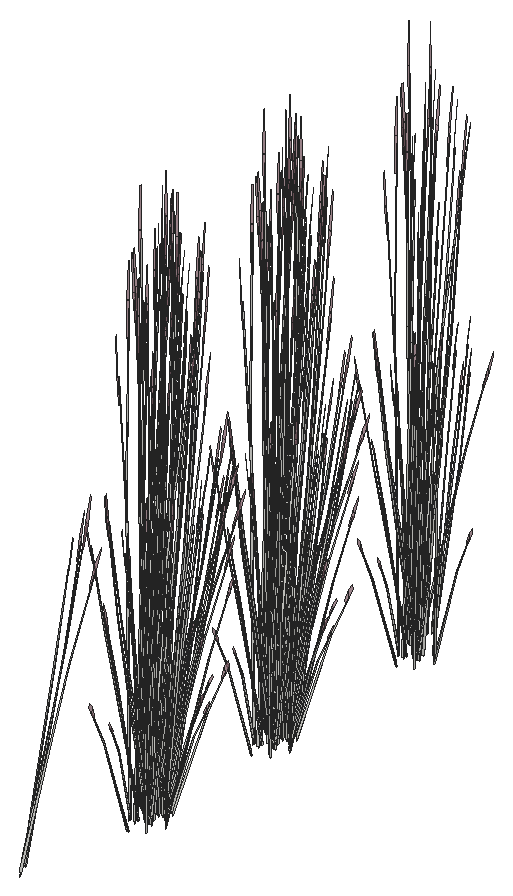
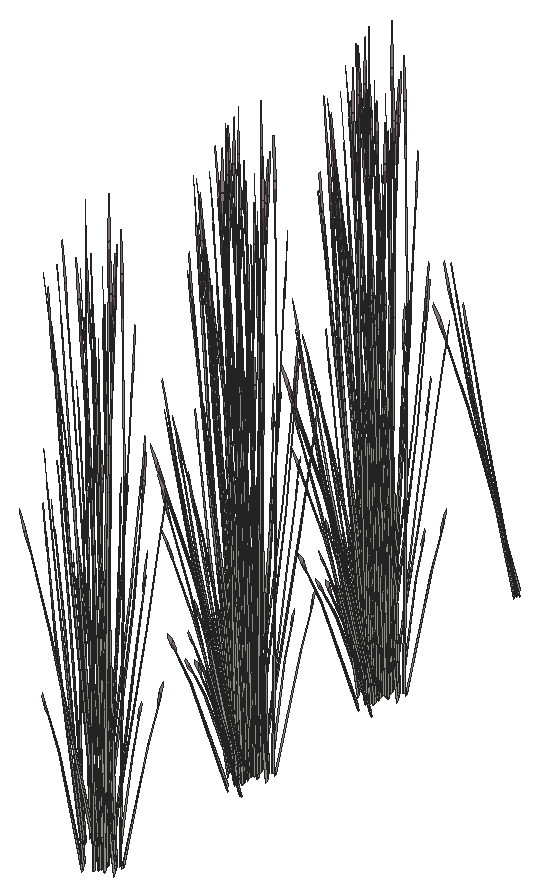
# SketchUp Ruby script. Lengths in inches.
U = 1.inch
M = Sketchup.active_model
def pt(a) = Geom::Point3d.new(a.map { |v| v * U })
def face(e, loops, mat)
  f = e.add_face(loops[0].map { |a| pt(a) })
  loops[1..].each { |l| e.add_face(l.map { |a| pt(a) }).erase! }
  f.material = f.back_material = mat if mat
  f
end
# faces: each face lists its corners as indices into pts; further lists are holes
def faces(e, pts, list, mat = nil) = list.each { |f| face(e, (f[0].is_a?(Array) ? f : [f]).map { |l| l.map { |i| pts[i] } }, mat) }
# xy, xz, yz: faces in a plane at the given z, y or x. An outline is a flat list of corners, or four numbers for a rectangle; further outlines are holes
def ring(l) = l.size == 4 ? [[l[0], l[1]], [l[2], l[1]], [l[2], l[3]], [l[0], l[3]]] : l.each_slice(2).to_a
def flat(e, list, mat, &to3) = list.each { |f| face(e, (f[0].is_a?(Array) ? f : [f]).map { |l| ring(l).map { |u, v| to3.(u, v) } }, mat) }
def xy(e, z, list, mat = nil) = flat(e, list, mat) { |x, y| [x, y, z] }
def xz(e, y, list, mat = nil) = flat(e, list, mat) { |x, z| [x, y, z] }
def yz(e, x, list, mat = nil) = flat(e, list, mat) { |y, z| [x, y, z] }
def lines(e, pts, list) = list.each { |a, b| e.add_line(pt(pts[a]), pt(pts[b])) }
# prism: a flat outline (further loops are holes) pulled along v
def prism(e, loops, v, mat = nil)
  f = face(e, loops, mat); d = Geom::Vector3d.new(v.map { |x| x * U })
  f.pushpull(f.normal.samedirection?(d) ? d.length : -d.length)
end
def box(e, o, s, mat = nil) = prism(e, [[o, [o[0] + s[0], o[1], o[2]], [o[0] + s[0], o[1] + s[1], o[2]], [o[0], o[1] + s[1], o[2]]]], [0, 0, s[2]], mat)
def at(x, y, z, deg = 0) = Geom::Transformation.translation(pt([x, y, z])) * Geom::Transformation.rotation(ORIGIN, Z_AXIS, deg.degrees)
def axes(o, x, y, z) = Geom::Transformation.new([*x, 0, *y, 0, *z, 0, *pt(o).to_a, 1])
def part(name) = M.definitions.add(name)
# library, detail: a bought-in or finely detailed component or shape, given as its bounding box
def library(name, o, s) = part(name).tap { |d| box(d.entities, o, s) }
def detail(e, o, s) = box(e.add_group.entities, o, s)
def put(e, d, t, mat = nil) = e.add_instance(d, t).tap { |i| i.material = mat if mat }
def group(e, t, mat = nil) = e.add_group.tap { |g| g.transformation = t; g.material = mat if mat }.entities
root = M.entities
M.materials.add("LightPink_Translucent").color = [144, 107, 117]
M.materials["LightPink_Translucent"].alpha = 0.75
c1 = part("blade")
p = [[2.15,0.21,22],[0,0.17,0],[0.09,0.45,0],[2.18,0.31,22],[2.29,0.31,22],[0.38,0.45,0],
  [2.48,0.24,33],[2.49,0.24,33],[2.48,0.22,33]]
faces(c1.entities,p,[[0,1,2,3],[4,5,2,3],[6,3,4,7],[8,0,3,6]])
c2 = part("seeds")
p = [[0.3,-0.1,1.38],[-0.01,-0.03,1.59],[-0.01,-0.03,0.03],[0.14,-0.07,-0.07],[0.29,-0.03,3],[0.15,0.01,3.11]]
faces(c2.entities,p,[[0,1,2,3],[1,0,4,5]],"LightPink_Translucent")
c3 = part("blade with seeds")
put(c3.entities,c1,at(0,0,0))
put(c3.entities,c2,axes([2.4,0.25,30.99],[1.5799,-0.05474,1.17369],[-0.12525,1.92788,0.29478],[-0.07173,-0.02425,1.56792]))
put(root,c3,axes([401.96,582.88,4.68],[0.34695,0.11691,-0.51099],[-0.11892,0.40083,-0.3958],[0.03181,0.16138,0.97773]))
put(root,c3,axes([402.16,582.05,3.875],[-0.08068,-0.14973,1.71376],[0.3728,-0.12606,0.13857],[0.08426,0.23506,0.73262]))
put(root,c3,axes([401.8,583.125,4.53],[-0.1064,0.35863,-0.35414],[-0.31043,-0.1046,0.4572],[0.02846,0.14439,0.87481]))
put(root,c3,axes([401.84,582.8,4.98],[0.16845,0.3792,-0.71045],[-0.34676,0.21133,0.08574],[0.03939,0.18322,1.00501]))
put(root,c3,axes([402.72,598.34,2.59],[-0.10032,0.0944,1.43002],[-0.30046,-0.16522,-0.30754],[0.05569,-0.20547,0.61141]))
put(root,c3,axes([401.98,597.83,1.49],[-0.0592,0.0168,1.76342],[-0.32738,-0.18913,-0.26939],[0.00549,-0.15776,0.30037]))
put(root,c3,axes([402.97,599.04,4.98],[0.00918,-0.43138,-0.71045],[0.38672,0.02897,0.08574],[0.04081,-0.18275,1.00501]))
put(root,c3,axes([402.3,598.35,4.53],[0.1064,-0.35863,-0.35414],[0.31043,0.1046,0.4572],[-0.02846,-0.14439,0.87481]))
put(root,c3,axes([402.53,598.82,3.875],[-0.06572,0.16029,1.71376],[-0.27569,-0.33172,0.13857],[0.12437,-0.20675,0.73262]))
put(root,c3,axes([402.35,597.59,2.77],[0.04528,0.27194,1.1486],[-0.25117,-0.15062,0.84392],[0.02703,-0.13924,0.25299]))
put(root,c3,axes([402.89,598.89,4.68],[-0.25266,-0.31335,-0.51099],[0.2669,-0.27442,-0.3958],[0.03844,-0.15921,0.97773]))
put(root,c3,axes([403.13,598.78,4.53],[0.23881,-0.24554,-0.35414],[0.22606,0.28036,0.4572],[0.0344,-0.14245,0.87481]))
put(root,c3,axes([403.43,598.63,1.49],[-0.05283,-0.03674,1.76342],[-0.13569,-0.41045,-0.26939],[0.09154,-0.11138,0.30037]))
put(root,c3,axes([403.42,599.79,4.98],[0.18436,-0.36797,-0.71045],[0.32306,0.26151,0.08574],[0.11008,-0.13332,1.00501]))
put(root,c3,axes([401.43,598.72,2.375],[-0.22066,-0.46731,0],[0.36918,-0.26061,-0.51607],[0.08408,-0.05936,1.63711]))
put(root,c3,axes([403.41,599.62,4.68],[-0.09067,-0.42583,-0.51099],[0.34336,-0.07449,-0.3958],[0.0984,-0.11438,0.97773]))
put(root,c3,axes([401.73,598.64,2.02],[0.33032,-0.23318,-0.49651],[0.19744,0.41812,0],[0.07523,-0.05311,1.57504]))
put(root,c3,axes([403.69,599.45,2.59],[-0.12609,-0.01381,1.43002],[-0.12917,-0.37055,-0.30754],[0.1549,-0.10482,0.61141]))
put(root,c3,axes([402.12,599.6,2.06],[0.23773,-0.35053,-0.62353],[0.29532,0.31785,-0.16365],[0.09526,-0.08744,1.37633]))
put(root,c3,axes([403.84,598.77,2.77],[-0.11756,0.2374,1.1486],[-0.10105,-0.31895,0.84392],[0.09709,-0.07992,0.25299]))
put(root,c3,axes([403.67,599.66,4.53],[0.30722,-0.06665,-0.35414],[0.08112,0.381,0.4572],[0.08804,-0.10234,0.87481]))
put(root,c3,axes([401.71,600.22,2.21],[0.17124,-0.42022,-0.44739],[0.35581,0.20224,0.21531],[0,-0.09687,1.43643]))
put(root,c3,axes([401.86,600.01,2.67],[-0.04113,-0.53214,-0.29095],[0.42835,-0.03218,-0.50002],[0.07543,-0.07088,1.59708]))
put(root,c3,axes([401.81,598.83,2.03],[0.32928,0.11539,-0.30978],[-0.08291,0.40636,0.30978],[0.06638,-0.04686,1.38974]))
put(root,c3,axes([401.92,600.42,2.43],[0.39767,0.22603,0.24065],[-0.19139,0.46966,0.50002],[0,-0.10827,1.60543]))
put(root,c3,axes([401.79,600.11,2.72],[-0.38326,0.02879,0.44739],[-0.03466,-0.47788,-0.21531],[0.06861,-0.04843,1.43643]))
put(root,c3,axes([403.57,600.5625,4.68],[0.09562,-0.42421,-0.51099],[0.32782,0.1454,-0.3958],[0.13199,-0.0389,0.97773]))
put(root,c3,axes([403.06,598.83,2.375],[0.22066,-0.46731,0],[0.36918,0.26061,-0.51607],[0.08408,0.05936,1.63711]))
put(root,c3,axes([401.78,600.28,2.36],[0.15345,0.52148,0.45755],[-0.43845,0.18134,0.17955],[0.00536,-0.09582,1.58856]))
put(root,c3,axes([403.92,600.68,1.98],[-0.22732,0.05597,1.41583],[-0.03618,-0.44548,0.08104],[0.15921,-0.06743,0.80566]))
put(root,c3,axes([404.34,600.29,2.26],[-0.21881,-0.29821,-0.06488],[0.23965,-0.27324,-0.29416],[0.0679,-0.01924,0.97024]))
put(root,c3,axes([402.33,600.33,2.21],[0,-0.53961,0],[0.44133,0,0],[0,0,1.79456]))
put(root,c3,axes([402.87,599.08,2.48],[-0.33032,-0.23318,0.49651],[0.19744,-0.41812,0],[0.07523,0.05311,1.57504]))
put(root,c3,axes([403.51,600.72,4.98],[0.31014,-0.20596,-0.71045],[0.17284,0.42397,0.08574],[0.14985,-0.04816,1.00501]))
put(root,c3,axes([402.12,599.99,2.36],[-0.29264,0.42323,0.45755],[-0.34767,-0.3736,0.17955],[0.07055,-0.04224,1.58856]))
put(root,c3,axes([401.61,599.29,2.47],[-0.10196,0.46348,0.17642],[-0.3731,-0.13116,0.35086],[0.06445,-0.00226,1.60407]))
put(root,c3,axes([401.46,599.66,1.59],[-0.3474,0.18671,1.28929],[-0.11057,-0.53572,0.50096],[0.21332,0.00891,1.46642]))
put(root,c3,axes([402.39,599.8,2.62],[0.06809,-0.4162,0.1448],[0.33266,0.07225,-0.41347],[0.06054,0.04274,1.26744]))
put(root,c3,axes([404.17,600.39,1.49],[-0.01845,-0.0708,1.76342],[0.12793,-0.41416,-0.26939],[0.12905,-0.00596,0.30037]))
put(root,c3,axes([402.25,599.91,2.72],[-0.21202,-0.39143,0.44739],[0.32115,-0.27564,-0.21531],[0.06861,0.04843,1.43643]))
put(root,c3,axes([402.36,599.9375,2.67],[0.35635,-0.30962,-0.29095],[0.23697,0.43749,-0.50002],[0.08792,0.04443,1.59708]))
put(root,c3,axes([403.78,600.76,4.53],[0.29332,0.1301,-0.35414],[-0.08555,0.37955,0.4572],[0.11809,-0.0348,0.87481]))
put(root,c3,axes([403.26,599.12,2.02],[0.33032,0.23318,-0.49651],[-0.19744,0.41812,0],[0.07523,0.05311,1.57504]))
put(root,c3,axes([402.63,600.45,2.21],[0.39487,0,0],[0,0.48281,0],[0,0,1.78407]))
put(root,c3,axes([402.74,599.3125,2.47],[-0.37926,0.12378,0.17642],[-0.09365,-0.46065,0.35086],[0.03382,0.06712,1.60407]))
put(root,c3,axes([402.98,600.29,3.875],[-0.14639,0.01056,1.71376],[0.09712,-0.45778,0.13857],[0.20862,0.02831,0.73262]))
put(root,c3,axes([403.17,599.29,2.03],[0.08291,0.40636,-0.30978],[-0.32928,0.11539,0.30978],[0.06638,0.04686,1.38974]))
put(root,c3,axes([402.5,600.2,2.38],[-0.44609,-0.09826,0.49198],[0.09078,-0.55493,0.19306],[0.06519,0.05359,1.70813]))
put(root,c3,axes([402.15,601.57,2.2],[-0.11516,-0.40207,0],[0.32884,-0.1408,0],[0,0,1.54371]))
put(root,c3,axes([402.58,601.51,2.18],[0.37054,-0.15823,-0.19198],[0.1302,0.45581,0.00008],[0.0409,-0.01749,1.73897]))
put(root,c3,axes([402.62,600.65,2.21],[0.24637,0.30123,0],[-0.24637,0.30123,0],[0,0,1.69266]))
put(root,c3,axes([403.29,600.52,2.47],[-0.2773,-0.3397,0.17642],[0.27945,-0.32949,0.35086],[-0.03063,0.06937,1.60407]))
put(root,c3,axes([402.78,600.01,2.06],[0.36714,0.07646,-0.62353],[-0.07747,0.47163,-0.16365],[0.10956,0.05715,1.37633]))
put(root,c3,axes([404.4,600.83,2.77],[-0.21807,0.07699,1.1486],[0.10265,-0.31819,0.84392],[0.11568,0.02177,0.25299]))
put(root,c3,axes([402.62,600.3,2.72],[0.17124,-0.42022,0.44739],[0.35581,0.20224,-0.21531],[0,0.09687,1.43643]))
put(root,c3,axes([402.55,600.54,2.29],[0,0.53934,-0.05637],[-0.44133,0,0],[0,0.01695,1.79368]))
put(root,c3,axes([402.58,600.16,2.21],[0.21202,0.39143,-0.44739],[-0.32115,0.27564,0.21531],[0.06861,0.04843,1.43643]))
put(root,c3,axes([404.02,601.8125,3.93],[-0.06755,-0.39203,-0.03492],[0.31928,-0.09013,-0.15832],[0.06667,0.02485,0.52218]))
put(root,c3,axes([403.52,600.53,2.48],[0,-0.46636,0.49651],[0.39487,0,0],[0,0.10622,1.57504]))
put(root,c3,axes([402.77,600.4,2.62],[0.32884,-0.136,0.1448],[0.11516,0.38837,-0.41347],[0,0.08547,1.26744]))
put(root,c3,axes([403.99,601.34,2.59],[-0.085,-0.1147,1.43002],[0.1106,-0.37943,-0.30754],[0.17198,0.0514,0.61141]))
put(root,c3,axes([402.47,601.76,2.2],[0.35581,0.20937,0],[-0.17124,0.43505,0],[0,0,1.74954]))
put(root,c3,axes([403.21,601.57,4.98],[0.35281,0.01123,-0.71045],[-0.0237,0.47284,0.08574],[0.14947,0.0499,1.00501]))
put(root,c3,axes([402.8125,601.95,2.48],[0.33032,-0.23318,0.49651],[0.19744,0.41812,0],[-0.07523,0.05311,1.57504]))
put(root,c3,axes([402.34,601.58,2.29],[0.15345,0.53576,-0.06012],[-0.43845,0.18773,0],[0.00536,0.01871,1.72173]))
put(root,c3,axes([403.78,600.61,2.375],[0.44133,0,0],[0,0.52122,-0.51607],[0,0.11871,1.63711]))
put(root,c3,axes([403.61,600.88,2.2],[-0.44111,-0.00373,-0.04976],[0,-0.52122,0.49943],[-0.01386,0.11865,1.58352]))
put(root,c3,axes([402.65,600.43,2.67],[0.39748,0.22252,-0.29095],[-0.19139,0.46966,-0.50002],[0.01249,0.11531,1.59708]))
put(root,c3,axes([403.42,601.77,4.53],[0.20082,0.29199,-0.35414],[-0.2293,0.2764,0.4572],[0.1165,0.04206,0.87481]))
put(root,c3,axes([403.52,600.96,2.03],[-0.24637,0.29097,-0.30978],[-0.24637,-0.29097,0.30978],[0,0.09372,1.38974]))
put(root,c3,axes([402.61,600.78,2.21],[-0.17124,0.42022,-0.44739],[-0.35581,-0.20224,0.21531],[0,0.09687,1.43643]))
put(root,c3,axes([402.62,601.98,2.33],[0.44186,0.15158,0.30756],[-0.11054,0.54181,-0.36492],[-0.07313,0.06781,1.64885]))
put(root,c3,axes([403.6875,600.97,2.02],[0,0.46636,-0.49651],[-0.39487,0,0],[0,0.10622,1.57504]))
put(root,c3,axes([402.7,601.02,3.875],[-0.1311,-0.08035,1.71376],[0.27131,-0.33708,0.13857],[0.16909,0.15206,0.73262]))
put(root,c3,axes([403.18,601.94,2.77],[-0.19872,-0.13409,1.1486],[0.2566,-0.13625,0.84392],[0.06921,0.11541,0.25299]))
put(root,c3,axes([403.24,602.43,1.49],[0.02571,-0.06733,1.76342],[0.32373,-0.19829,-0.26939],[0.09815,0.10263,0.30037]))
put(root,c3,axes([402.8125,600.9,2.09],[0.12941,0.42699,-0.69212],[-0.37279,0.15378,-0.18165],[0.0143,0.14459,1.52773]))
put(root,c3,axes([402.74,602.12,4.68],[0.34827,-0.11086,-0.51099],[0.06092,0.41983,-0.3958],[0.09354,0.12031,0.97773]))
put(root,c3,axes([403.22,602.55,2.67],[-0.22633,-0.01463,1.0506],[0.14947,-0.31064,0.58006],[0.08941,0.11036,0.8241]))
put(root,c3,axes([402.48,601.79,2.59],[0.00623,-0.15459,1.43002],[0.29764,-0.17268,-0.30754],[0.09188,0.18503,0.61141]))
put(root,c3,axes([401.73,602.42,1.49],[0.05712,-0.02538,1.76342],[0.34359,0.13968,-0.26939],[0.01005,0.15742,0.30037]))
put(root,c3,axes([401.96,602.31,4.68],[0.34695,0.11691,-0.51099],[-0.11892,0.40083,-0.3958],[0.03181,0.16138,0.97773]))
put(root,c3,axes([402.16,601.49,3.875],[-0.08068,-0.14973,1.71376],[0.3728,-0.12606,0.13857],[0.08426,0.23506,0.73262]))
put(root,c3,axes([401.8,602.5625,4.53],[-0.1064,0.35863,-0.35414],[-0.31043,-0.1046,0.4572],[0.02846,0.14439,0.87481]))
put(root,c3,axes([401.84,602.24,4.98],[0.16845,0.3792,-0.71045],[-0.34676,0.21133,0.08574],[0.03939,0.18322,1.00501]))
put(root,c3,axes([402.72,615.92,2.59],[-0.10032,0.0944,1.43002],[-0.30046,-0.16522,-0.30754],[0.05569,-0.20547,0.61141]))
put(root,c3,axes([401.98,615.41,1.49],[-0.0592,0.0168,1.76342],[-0.32738,-0.18913,-0.26939],[0.00549,-0.15776,0.30037]))
put(root,c3,axes([402.97,616.62,4.98],[0.00918,-0.43138,-0.71045],[0.38672,0.02897,0.08574],[0.04081,-0.18275,1.00501]))
put(root,c3,axes([402.3,615.93,4.53],[0.1064,-0.35863,-0.35414],[0.31043,0.1046,0.4572],[-0.02846,-0.14439,0.87481]))
put(root,c3,axes([402.53,616.4,3.875],[-0.06572,0.16029,1.71376],[-0.27569,-0.33172,0.13857],[0.12437,-0.20675,0.73262]))
put(root,c3,axes([402.35,615.17,2.77],[0.04528,0.27194,1.1486],[-0.25117,-0.15062,0.84392],[0.02703,-0.13924,0.25299]))
put(root,c3,axes([402.89,616.48,4.68],[-0.25266,-0.31335,-0.51099],[0.2669,-0.27442,-0.3958],[0.03844,-0.15921,0.97773]))
put(root,c3,axes([403.13,616.36,4.53],[0.23881,-0.24554,-0.35414],[0.22606,0.28036,0.4572],[0.0344,-0.14245,0.87481]))
put(root,c3,axes([403.43,616.21,1.49],[-0.05283,-0.03674,1.76342],[-0.13569,-0.41045,-0.26939],[0.09154,-0.11138,0.30037]))
put(root,c3,axes([403.42,617.37,4.98],[0.18436,-0.36797,-0.71045],[0.32306,0.26151,0.08574],[0.11008,-0.13332,1.00501]))
put(root,c3,axes([401.43,616.3,2.375],[-0.22066,-0.46731,0],[0.36918,-0.26061,-0.51607],[0.08408,-0.05936,1.63711]))
put(root,c3,axes([403.41,617.2,4.68],[-0.09067,-0.42583,-0.51099],[0.34336,-0.07449,-0.3958],[0.0984,-0.11438,0.97773]))
put(root,c3,axes([401.73,616.23,2.02],[0.33032,-0.23318,-0.49651],[0.19744,0.41812,0],[0.07523,-0.05311,1.57504]))
put(root,c3,axes([403.69,617.03,2.59],[-0.12609,-0.01381,1.43002],[-0.12917,-0.37055,-0.30754],[0.1549,-0.10482,0.61141]))
put(root,c3,axes([402.12,617.18,2.06],[0.23773,-0.35053,-0.62353],[0.29532,0.31785,-0.16365],[0.09526,-0.08744,1.37633]))
put(root,c3,axes([403.84,616.35,2.77],[-0.11756,0.2374,1.1486],[-0.10105,-0.31895,0.84392],[0.09709,-0.07992,0.25299]))
put(root,c3,axes([403.67,617.24,4.53],[0.30722,-0.06665,-0.35414],[0.08112,0.381,0.4572],[0.08804,-0.10234,0.87481]))
put(root,c3,axes([401.71,617.8,2.21],[0.17124,-0.42022,-0.44739],[0.35581,0.20224,0.21531],[0,-0.09687,1.43643]))
put(root,c3,axes([401.86,617.59,2.67],[-0.04113,-0.53214,-0.29095],[0.42835,-0.03218,-0.50002],[0.07543,-0.07088,1.59708]))
put(root,c3,axes([401.81,616.41,2.03],[0.32928,0.11539,-0.30978],[-0.08291,0.40636,0.30978],[0.06638,-0.04686,1.38974]))
put(root,c3,axes([401.92,618.01,2.43],[0.39767,0.22603,0.24065],[-0.19139,0.46966,0.50002],[0,-0.10827,1.60543]))
put(root,c3,axes([401.79,617.69,2.72],[-0.38326,0.02879,0.44739],[-0.03466,-0.47788,-0.21531],[0.06861,-0.04843,1.43643]))
put(root,c3,axes([403.57,618.14,4.68],[0.09562,-0.42421,-0.51099],[0.32782,0.1454,-0.3958],[0.13199,-0.0389,0.97773]))
put(root,c3,axes([403.06,616.42,2.375],[0.22066,-0.46731,0],[0.36918,0.26061,-0.51607],[0.08408,0.05936,1.63711]))
put(root,c3,axes([401.78,617.86,2.36],[0.15345,0.52148,0.45755],[-0.43845,0.18134,0.17955],[0.00536,-0.09582,1.58856]))
put(root,c3,axes([403.92,618.26,1.98],[-0.22732,0.05597,1.41583],[-0.03618,-0.44548,0.08104],[0.15921,-0.06743,0.80566]))
put(root,c3,axes([404.34,617.87,2.26],[-0.21881,-0.29821,-0.06488],[0.23965,-0.27324,-0.29416],[0.0679,-0.01924,0.97024]))
put(root,c3,axes([402.33,617.91,2.21],[0,-0.53961,0],[0.44133,0,0],[0,0,1.79456]))
put(root,c3,axes([402.87,616.66,2.48],[-0.33032,-0.23318,0.49651],[0.19744,-0.41812,0],[0.07523,0.05311,1.57504]))
put(root,c3,axes([403.51,618.3,4.98],[0.31014,-0.20596,-0.71045],[0.17284,0.42397,0.08574],[0.14985,-0.04816,1.00501]))
put(root,c3,axes([402.12,617.57,2.36],[-0.29264,0.42323,0.45755],[-0.34767,-0.3736,0.17955],[0.07055,-0.04224,1.58856]))
put(root,c3,axes([401.61,616.87,2.47],[-0.10196,0.46348,0.17642],[-0.3731,-0.13116,0.35086],[0.06445,-0.00226,1.60407]))
put(root,c3,axes([401.46,617.25,1.59],[-0.3474,0.18671,1.28929],[-0.11057,-0.53572,0.50096],[0.21332,0.00891,1.46642]))
put(root,c3,axes([402.39,617.39,2.62],[0.06809,-0.4162,0.1448],[0.33266,0.07225,-0.41347],[0.06054,0.04274,1.26744]))
put(root,c3,axes([404.17,617.97,1.49],[-0.01845,-0.0708,1.76342],[0.12793,-0.41416,-0.26939],[0.12905,-0.00596,0.30037]))
put(root,c3,axes([402.25,617.5,2.72],[-0.21202,-0.39143,0.44739],[0.32115,-0.27564,-0.21531],[0.06861,0.04843,1.43643]))
put(root,c3,axes([402.36,617.52,2.67],[0.35635,-0.30962,-0.29095],[0.23697,0.43749,-0.50002],[0.08792,0.04443,1.59708]))
put(root,c3,axes([403.78,618.34,4.53],[0.29332,0.1301,-0.35414],[-0.08555,0.37955,0.4572],[0.11809,-0.0348,0.87481]))
put(root,c3,axes([403.26,616.7,2.02],[0.33032,0.23318,-0.49651],[-0.19744,0.41812,0],[0.07523,0.05311,1.57504]))
put(root,c3,axes([402.63,618.03,2.21],[0.39487,0,0],[0,0.48281,0],[0,0,1.78407]))
put(root,c3,axes([402.74,616.9,2.47],[-0.37926,0.12378,0.17642],[-0.09365,-0.46065,0.35086],[0.03382,0.06712,1.60407]))
put(root,c3,axes([402.98,617.87,3.875],[-0.14639,0.01056,1.71376],[0.09712,-0.45778,0.13857],[0.20862,0.02831,0.73262]))
put(root,c3,axes([403.17,616.87,2.03],[0.08291,0.40636,-0.30978],[-0.32928,0.11539,0.30978],[0.06638,0.04686,1.38974]))
put(root,c3,axes([402.5,617.78,2.38],[-0.44609,-0.09826,0.49198],[0.09078,-0.55493,0.19306],[0.06519,0.05359,1.70813]))
put(root,c3,axes([402.15,619.15,2.2],[-0.11516,-0.40207,0],[0.32884,-0.1408,0],[0,0,1.54371]))
put(root,c3,axes([402.58,619.1,2.18],[0.37054,-0.15823,-0.19198],[0.1302,0.45581,0.00008],[0.0409,-0.01749,1.73897]))
put(root,c3,axes([402.62,618.24,2.21],[0.24637,0.30123,0],[-0.24637,0.30123,0],[0,0,1.69266]))
put(root,c3,axes([403.29,618.1,2.47],[-0.2773,-0.3397,0.17642],[0.27945,-0.32949,0.35086],[-0.03063,0.06937,1.60407]))
put(root,c3,axes([402.78,617.59,2.06],[0.36714,0.07646,-0.62353],[-0.07747,0.47163,-0.16365],[0.10956,0.05715,1.37633]))
put(root,c3,axes([404.4,618.42,2.77],[-0.21807,0.07699,1.1486],[0.10265,-0.31819,0.84392],[0.11568,0.02177,0.25299]))
put(root,c3,axes([402.62,617.88,2.72],[0.17124,-0.42022,0.44739],[0.35581,0.20224,-0.21531],[0,0.09687,1.43643]))
put(root,c3,axes([402.55,618.125,2.29],[0,0.53934,-0.05637],[-0.44133,0,0],[0,0.01695,1.79368]))
put(root,c3,axes([402.58,617.74,2.21],[0.21202,0.39143,-0.44739],[-0.32115,0.27564,0.21531],[0.06861,0.04843,1.43643]))
put(root,c3,axes([404.02,619.4,3.93],[-0.06755,-0.39203,-0.03492],[0.31928,-0.09013,-0.15832],[0.06667,0.02485,0.52218]))
put(root,c3,axes([403.52,618.12,2.48],[0,-0.46636,0.49651],[0.39487,0,0],[0,0.10622,1.57504]))
put(root,c3,axes([402.77,617.98,2.62],[0.32884,-0.136,0.1448],[0.11516,0.38837,-0.41347],[0,0.08547,1.26744]))
put(root,c3,axes([403.99,618.93,2.59],[-0.085,-0.1147,1.43002],[0.1106,-0.37943,-0.30754],[0.17198,0.0514,0.61141]))
put(root,c3,axes([402.47,619.34,2.2],[0.35581,0.20937,0],[-0.17124,0.43505,0],[0,0,1.74954]))
put(root,c3,axes([403.21,619.16,4.98],[0.35281,0.01123,-0.71045],[-0.0237,0.47284,0.08574],[0.14947,0.0499,1.00501]))
put(root,c3,axes([402.8125,619.54,2.48],[0.33032,-0.23318,0.49651],[0.19744,0.41812,0],[-0.07523,0.05311,1.57504]))
put(root,c3,axes([402.34,619.17,2.29],[0.15345,0.53576,-0.06012],[-0.43845,0.18773,0],[0.00536,0.01871,1.72173]))
put(root,c3,axes([403.78,618.2,2.375],[0.44133,0,0],[0,0.52122,-0.51607],[0,0.11871,1.63711]))
put(root,c3,axes([403.61,618.46,2.2],[-0.44111,-0.00373,-0.04976],[0,-0.52122,0.49943],[-0.01386,0.11865,1.58352]))
put(root,c3,axes([402.65,618.01,2.67],[0.39748,0.22252,-0.29095],[-0.19139,0.46966,-0.50002],[0.01249,0.11531,1.59708]))
put(root,c3,axes([403.42,619.35,4.53],[0.20082,0.29199,-0.35414],[-0.2293,0.2764,0.4572],[0.1165,0.04206,0.87481]))
put(root,c3,axes([403.52,618.54,2.03],[-0.24637,0.29097,-0.30978],[-0.24637,-0.29097,0.30978],[0,0.09372,1.38974]))
put(root,c3,axes([402.61,618.36,2.21],[-0.17124,0.42022,-0.44739],[-0.35581,-0.20224,0.21531],[0,0.09687,1.43643]))
put(root,c3,axes([402.62,619.57,2.33],[0.44186,0.15158,0.30756],[-0.11054,0.54181,-0.36492],[-0.07313,0.06781,1.64885]))
put(root,c3,axes([403.6875,618.55,2.02],[0,0.46636,-0.49651],[-0.39487,0,0],[0,0.10622,1.57504]))
put(root,c3,axes([402.7,618.6,3.875],[-0.1311,-0.08035,1.71376],[0.27131,-0.33708,0.13857],[0.16909,0.15206,0.73262]))
put(root,c3,axes([403.18,619.52,2.77],[-0.19872,-0.13409,1.1486],[0.2566,-0.13625,0.84392],[0.06921,0.11541,0.25299]))
put(root,c3,axes([403.24,620.02,1.49],[0.02571,-0.06733,1.76342],[0.32373,-0.19829,-0.26939],[0.09815,0.10263,0.30037]))
put(root,c3,axes([402.8125,618.49,2.09],[0.12941,0.42699,-0.69212],[-0.37279,0.15378,-0.18165],[0.0143,0.14459,1.52773]))
put(root,c3,axes([402.74,619.7,4.68],[0.34827,-0.11086,-0.51099],[0.06092,0.41983,-0.3958],[0.09354,0.12031,0.97773]))
put(root,c3,axes([403.22,620.13,2.67],[-0.22633,-0.01463,1.0506],[0.14947,-0.31064,0.58006],[0.08941,0.11036,0.8241]))
put(root,c3,axes([402.48,619.375,2.59],[0.00623,-0.15459,1.43002],[0.29764,-0.17268,-0.30754],[0.09188,0.18503,0.61141]))
put(root,c3,axes([401.73,620,1.49],[0.05712,-0.02538,1.76342],[0.34359,0.13968,-0.26939],[0.01005,0.15742,0.30037]))
put(root,c3,axes([401.96,619.9,4.68],[0.34695,0.11691,-0.51099],[-0.11892,0.40083,-0.3958],[0.03181,0.16138,0.97773]))
put(root,c3,axes([402.16,619.07,3.875],[-0.08068,-0.14973,1.71376],[0.3728,-0.12606,0.13857],[0.08426,0.23506,0.73262]))
put(root,c3,axes([401.8,620.14,4.53],[-0.1064,0.35863,-0.35414],[-0.31043,-0.1046,0.4572],[0.02846,0.14439,0.87481]))
put(root,c3,axes([401.84,619.82,4.98],[0.16845,0.3792,-0.71045],[-0.34676,0.21133,0.08574],[0.03939,0.18322,1.00501]))
put(root,c3,axes([402.72,636.46,2.59],[-0.10032,0.0944,1.43002],[-0.30046,-0.16522,-0.30754],[0.05569,-0.20547,0.61141]))
put(root,c3,axes([401.98,635.94,1.49],[-0.0592,0.0168,1.76342],[-0.32738,-0.18913,-0.26939],[0.00549,-0.15776,0.30037]))
put(root,c3,axes([402.97,637.16,4.98],[0.00918,-0.43138,-0.71045],[0.38672,0.02897,0.08574],[0.04081,-0.18275,1.00501]))
put(root,c3,axes([402.3,636.46,4.53],[0.1064,-0.35863,-0.35414],[0.31043,0.1046,0.4572],[-0.02846,-0.14439,0.87481]))
put(root,c3,axes([402.53,636.9375,3.875],[-0.06572,0.16029,1.71376],[-0.27569,-0.33172,0.13857],[0.12437,-0.20675,0.73262]))
put(root,c3,axes([402.35,635.71,2.77],[0.04528,0.27194,1.1486],[-0.25117,-0.15062,0.84392],[0.02703,-0.13924,0.25299]))
put(root,c3,axes([402.89,637.01,4.68],[-0.25266,-0.31335,-0.51099],[0.2669,-0.27442,-0.3958],[0.03844,-0.15921,0.97773]))
put(root,c3,axes([403.13,636.9,4.53],[0.23881,-0.24554,-0.35414],[0.22606,0.28036,0.4572],[0.0344,-0.14245,0.87481]))
put(root,c3,axes([403.43,636.75,1.49],[-0.05283,-0.03674,1.76342],[-0.13569,-0.41045,-0.26939],[0.09154,-0.11138,0.30037]))
put(root,c3,axes([403.42,637.91,4.98],[0.18436,-0.36797,-0.71045],[0.32306,0.26151,0.08574],[0.11008,-0.13332,1.00501]))
put(root,c3,axes([401.43,636.83,2.375],[-0.22066,-0.46731,0],[0.36918,-0.26061,-0.51607],[0.08408,-0.05936,1.63711]))
put(root,c3,axes([403.41,637.73,4.68],[-0.09067,-0.42583,-0.51099],[0.34336,-0.07449,-0.3958],[0.0984,-0.11438,0.97773]))
put(root,c3,axes([401.73,636.76,2.02],[0.33032,-0.23318,-0.49651],[0.19744,0.41812,0],[0.07523,-0.05311,1.57504]))
put(root,c3,axes([403.69,637.57,2.59],[-0.12609,-0.01381,1.43002],[-0.12917,-0.37055,-0.30754],[0.1549,-0.10482,0.61141]))
put(root,c3,axes([402.12,637.72,2.06],[0.23773,-0.35053,-0.62353],[0.29532,0.31785,-0.16365],[0.09526,-0.08744,1.37633]))
put(root,c3,axes([403.84,636.89,2.77],[-0.11756,0.2374,1.1486],[-0.10105,-0.31895,0.84392],[0.09709,-0.07992,0.25299]))
put(root,c3,axes([403.67,637.78,4.53],[0.30722,-0.06665,-0.35414],[0.08112,0.381,0.4572],[0.08804,-0.10234,0.87481]))
put(root,c3,axes([401.71,638.33,2.21],[0.17124,-0.42022,-0.44739],[0.35581,0.20224,0.21531],[0,-0.09687,1.43643]))
put(root,c3,axes([401.86,638.125,2.67],[-0.04113,-0.53214,-0.29095],[0.42835,-0.03218,-0.50002],[0.07543,-0.07088,1.59708]))
put(root,c3,axes([401.81,636.95,2.03],[0.32928,0.11539,-0.30978],[-0.08291,0.40636,0.30978],[0.06638,-0.04686,1.38974]))
put(root,c3,axes([401.92,638.54,2.43],[0.39767,0.22603,0.24065],[-0.19139,0.46966,0.50002],[0,-0.10827,1.60543]))
put(root,c3,axes([401.79,638.23,2.72],[-0.38326,0.02879,0.44739],[-0.03466,-0.47788,-0.21531],[0.06861,-0.04843,1.43643]))
put(root,c3,axes([403.57,638.68,4.68],[0.09562,-0.42421,-0.51099],[0.32782,0.1454,-0.3958],[0.13199,-0.0389,0.97773]))
put(root,c3,axes([403.06,636.95,2.375],[0.22066,-0.46731,0],[0.36918,0.26061,-0.51607],[0.08408,0.05936,1.63711]))
put(root,c3,axes([401.78,638.4,2.36],[0.15345,0.52148,0.45755],[-0.43845,0.18134,0.17955],[0.00536,-0.09582,1.58856]))
put(root,c3,axes([403.92,638.8,1.98],[-0.22732,0.05597,1.41583],[-0.03618,-0.44548,0.08104],[0.15921,-0.06743,0.80566]))
put(root,c3,axes([404.34,638.4,2.26],[-0.21881,-0.29821,-0.06488],[0.23965,-0.27324,-0.29416],[0.0679,-0.01924,0.97024]))
put(root,c3,axes([402.33,638.44,2.21],[0,-0.53961,0],[0.44133,0,0],[0,0,1.79456]))
put(root,c3,axes([402.87,637.2,2.48],[-0.33032,-0.23318,0.49651],[0.19744,-0.41812,0],[0.07523,0.05311,1.57504]))
put(root,c3,axes([403.51,638.83,4.98],[0.31014,-0.20596,-0.71045],[0.17284,0.42397,0.08574],[0.14985,-0.04816,1.00501]))
put(root,c3,axes([402.12,638.1,2.36],[-0.29264,0.42323,0.45755],[-0.34767,-0.3736,0.17955],[0.07055,-0.04224,1.58856]))
put(root,c3,axes([401.61,637.41,2.47],[-0.10196,0.46348,0.17642],[-0.3731,-0.13116,0.35086],[0.06445,-0.00226,1.60407]))
put(root,c3,axes([401.46,637.78,1.59],[-0.3474,0.18671,1.28929],[-0.11057,-0.53572,0.50096],[0.21332,0.00891,1.46642]))
put(root,c3,axes([402.39,637.92,2.62],[0.06809,-0.4162,0.1448],[0.33266,0.07225,-0.41347],[0.06054,0.04274,1.26744]))
put(root,c3,axes([404.17,638.51,1.49],[-0.01845,-0.0708,1.76342],[0.12793,-0.41416,-0.26939],[0.12905,-0.00596,0.30037]))
put(root,c3,axes([402.25,638.03,2.72],[-0.21202,-0.39143,0.44739],[0.32115,-0.27564,-0.21531],[0.06861,0.04843,1.43643]))
put(root,c3,axes([402.36,638.06,2.67],[0.35635,-0.30962,-0.29095],[0.23697,0.43749,-0.50002],[0.08792,0.04443,1.59708]))
put(root,c3,axes([403.78,638.87,4.53],[0.29332,0.1301,-0.35414],[-0.08555,0.37955,0.4572],[0.11809,-0.0348,0.87481]))
put(root,c3,axes([403.26,637.23,2.02],[0.33032,0.23318,-0.49651],[-0.19744,0.41812,0],[0.07523,0.05311,1.57504]))
put(root,c3,axes([402.63,638.5625,2.21],[0.39487,0,0],[0,0.48281,0],[0,0,1.78407]))
put(root,c3,axes([402.74,637.43,2.47],[-0.37926,0.12378,0.17642],[-0.09365,-0.46065,0.35086],[0.03382,0.06712,1.60407]))
put(root,c3,axes([402.98,638.4,3.875],[-0.14639,0.01056,1.71376],[0.09712,-0.45778,0.13857],[0.20862,0.02831,0.73262]))
put(root,c3,axes([403.17,637.41,2.03],[0.08291,0.40636,-0.30978],[-0.32928,0.11539,0.30978],[0.06638,0.04686,1.38974]))
